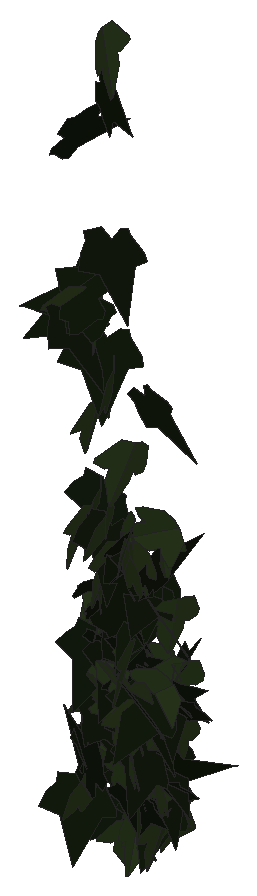
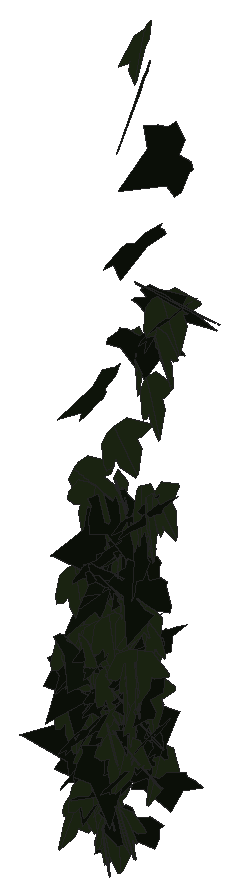
# SketchUp Ruby script. Lengths in inches.
U = 1.inch
M = Sketchup.active_model
def pt(a) = Geom::Point3d.new(a.map { |v| v * U })
def face(e, loops, mat)
  f = e.add_face(loops[0].map { |a| pt(a) })
  loops[1..].each { |l| e.add_face(l.map { |a| pt(a) }).erase! }
  f.material = f.back_material = mat if mat
  f
end
# faces: each face lists its corners as indices into pts; further lists are holes
def faces(e, pts, list, mat = nil) = list.each { |f| face(e, (f[0].is_a?(Array) ? f : [f]).map { |l| l.map { |i| pts[i] } }, mat) }
# xy, xz, yz: faces in a plane at the given z, y or x. An outline is a flat list of corners, or four numbers for a rectangle; further outlines are holes
def ring(l) = l.size == 4 ? [[l[0], l[1]], [l[2], l[1]], [l[2], l[3]], [l[0], l[3]]] : l.each_slice(2).to_a
def flat(e, list, mat, &to3) = list.each { |f| face(e, (f[0].is_a?(Array) ? f : [f]).map { |l| ring(l).map { |u, v| to3.(u, v) } }, mat) }
def xy(e, z, list, mat = nil) = flat(e, list, mat) { |x, y| [x, y, z] }
def xz(e, y, list, mat = nil) = flat(e, list, mat) { |x, z| [x, y, z] }
def yz(e, x, list, mat = nil) = flat(e, list, mat) { |y, z| [x, y, z] }
def lines(e, pts, list) = list.each { |a, b| e.add_line(pt(pts[a]), pt(pts[b])) }
# prism: a flat outline (further loops are holes) pulled along v
def prism(e, loops, v, mat = nil)
  f = face(e, loops, mat); d = Geom::Vector3d.new(v.map { |x| x * U })
  f.pushpull(f.normal.samedirection?(d) ? d.length : -d.length)
end
def box(e, o, s, mat = nil) = prism(e, [[o, [o[0] + s[0], o[1], o[2]], [o[0] + s[0], o[1] + s[1], o[2]], [o[0], o[1] + s[1], o[2]]]], [0, 0, s[2]], mat)
def at(x, y, z, deg = 0) = Geom::Transformation.translation(pt([x, y, z])) * Geom::Transformation.rotation(ORIGIN, Z_AXIS, deg.degrees)
def axes(o, x, y, z) = Geom::Transformation.new([*x, 0, *y, 0, *z, 0, *pt(o).to_a, 1])
def part(name) = M.definitions.add(name)
# library, detail: a bought-in or finely detailed component or shape, given as its bounding box
def library(name, o, s) = part(name).tap { |d| box(d.entities, o, s) }
def detail(e, o, s) = box(e.add_group.entities, o, s)
def put(e, d, t, mat = nil) = e.add_instance(d, t).tap { |i| i.material = mat if mat }
def group(e, t, mat = nil) = e.add_group.tap { |g| g.transformation = t; g.material = mat if mat }.entities
root = M.entities
M.materials.add("efeu1").color = [18, 25, 13]
M.materials.add("efeu2").color = [43, 57, 29]
c1 = part("ivyleaf_10")
p = [[0,0.5,-0.03],[-0.0625,2.02,-0.43],[-0.19,2.01,-0.46],[-0.54,1.05,-0.29],[-0.52,0.625,-0.18],[-0.83,0.76,-0.28],
  [-1.16,0.64,-0.33],[-1.15,0.33,-0.24],[-0.77,-0.39,0.02],[-0.3,-0.51,0.16],[0.04,-0.48,0.23],[-0.02,2.01,-0.4375],
  [-0.06,2.01,-0.43],[0.04,-0.49,0.23],[0.67,-0.49,0.14],[1.38,0.36,-0.2],[1.375,0.51,-0.24],[0.81,0.65,-0.19],
  [0.62,0.59,-0.15],[0.6,1.09,-0.28],[0.5,1.23,-0.31]]
faces(c1.entities,p,[[0,1,2,3,4,5,6,7,8,9,10],[11,12,0,13,14,15,16,17,18,19,20]],"efeu2")
c2 = part("ivyleaf_9")
p = [[1.54,2.16,1.25],[1.36,2.04,1.19],[-0.21,0.99,0.68],[-0.71,1.11,0.82],[-0.85,0.86,0.67],[-0.8,0.17,0.21],
  [-0.9,-0.01,0.1],[-0.67,-0.16,-0.02],[-0.08,-0.08,-0.05],[-0.03,-0.6,-0.4],[0.65,-0.88,-0.66],[0.83,-0.6,-0.49],
  [1.29,-0.42,-0.43],[1.8125,-0.07,-0.26],[1.21,0.44,0.15]]
faces(c2.entities,p,[[0,1,2,3,4,5,6,7,8,9,10,11,12,13,14]],"efeu1")
put(root,c1,axes([541.64,132.27,226.93],[-0.32026,-0.86998,0.20243],[-0.08974,-0.18262,-0.92683],[0.8887,-0.33195,-0.02065]))
put(root,c1,axes([541.54,132.71,225.9],[0.78925,-0.47005,-0.20203],[-0.14106,0.15709,-0.91657],[0.49179,0.79941,0.06132]))
put(root,c2,axes([541.35,132.85,207.7],[-0.47891,-0.67172,-0.25991],[0.19866,0.17682,-0.82303],[0.69231,-0.5154,0.05637]))
put(root,c1,axes([541.64,133.93,212.93],[-0.72073,-0.4905,0.00951],[0.0309,-0.06226,-0.86908],[0.48961,-0.7181,0.06886]))
put(root,c1,axes([541.52,134.76,206.88],[0.64822,-0.5421,0.01637],[0.01224,-0.01088,-0.84502],[0.5422,0.64834,-0.00049]))
put(root,c1,axes([541.65,133.19,211.51],[-0.09073,-0.85028,-0.01671],[0.00087,0.01671,-0.85511],[0.85045,-0.09073,-0.0009]))
put(root,c2,axes([541.25,133.23,209.89],[0.53426,-0.47664,-0.49908],[-0.2064,0.49191,-0.69074],[0.65853,0.54087,0.18841]))
put(root,c1,axes([541.63,133.15,218.88],[0.36674,-0.81694,-0.21878],[-0.0264,0.22729,-0.89297],[0.84532,0.36153,0.06703]))
put(root,c1,axes([541.69,133.99,210.95],[-0.3938,0.77477,0.0623],[-0.19432,-0.03052,-0.84884],[-0.75258,-0.39752,0.18658]))
put(root,c1,axes([541.23,133.61,214.32],[0.7081,-0.28038,0.42554],[0.41728,-0.09916,-0.7597],[0.29252,0.82016,0.05362]))
put(root,c2,axes([541.73,133.15,215.86],[0.28251,0.81104,0.16092],[-0.02124,0.17712,-0.85538],[-0.82658,0.27264,0.07698]))
put(root,c2,axes([541.42,131.87,233.13],[0.36103,0.55969,0.69828],[0.40169,0.57149,-0.66576],[-0.79968,0.53975,-0.01917]))
put(root,c1,axes([541.7,134.55,209.64],[-0.83966,-0.17869,-0.05465],[0.05299,0.01358,-0.85846],[0.17919,-0.84133,-0.00224]))
put(root,c2,axes([542.4,132.08,227.21],[-0.77918,0.34542,0.40853],[-0.47121,-0.10136,-0.81303],[-0.25332,-0.87393,0.25577]))
put(root,c1,axes([541.74,132.3125,208.3],[-0.04652,-0.72628,-0.52307],[0.05961,0.5201,-0.72746],[0.89304,-0.07255,0.02131]))
put(root,c2,axes([541.58,133.1875,208.68],[0.08281,-0.22127,0.85612],[0.45325,0.74893,0.14972],[-0.75925,0.42296,0.18276]))
put(root,c2,axes([542.27,132.29,227.06],[-0.86557,-0.19065,0.32604],[-0.31473,-0.08657,-0.88618],[0.20879,-0.92088,0.01581]))
put(root,c1,axes([541.81,133.7,212.51],[0.45582,-0.73664,-0.18739],[-0.00413,0.2161,-0.85954],[0.76009,0.44293,0.10771]))
put(root,c2,axes([541.36,134.35,206.7],[-0.10384,-0.39536,-0.73817],[0.38567,0.63766,-0.39578],[0.74328,-0.3861,0.10223]))
put(root,c2,axes([541.61,133.67,218.73],[-0.199,-0.81888,0.29676],[0.03297,-0.31127,-0.83681],[0.87037,-0.17544,0.09955]))
put(root,c2,axes([541.71,133.16,213.27],[-0.26657,-0.81591,0.24377],[-0.01935,-0.24957,-0.85646],[0.85133,-0.26115,0.05686]))
put(root,c2,axes([541.38,133.9375,209.84],[0.83919,-0.16882,0.03563],[0.03189,-0.02215,-0.85586],[0.16956,0.83965,-0.01541]))
put(root,c1,axes([541.96,133.86,212.31],[0.10595,-0.78561,-0.3752],[-0.01939,0.37575,-0.79222],[0.87039,0.104,0.02802]))
put(root,c2,axes([542.2,134.16,209.66],[-0.80552,0.2288,-0.18474],[0.16416,-0.09712,-0.83604],[-0.24399,-0.8207,0.04743]))
put(root,c2,axes([541.53,134.37,208.58],[0.18246,-0.80067,-0.25157],[0.00667,0.25883,-0.81891],[0.83923,0.17202,0.06121]))
put(root,c1,axes([541.82,134.63,206.85],[0.83582,-0.05974,-0.04926],[-0.0495,-0.00152,-0.83794],[0.05955,0.83727,-0.00503]))
put(root,c1,axes([541.52,133.75,214.92],[0.68119,0.29451,0.46585],[0.32645,0.38113,-0.7183],[-0.44406,0.73197,0.18657]))
put(root,c1,axes([541.91,132.17,218.6875],[0.25139,-0.80054,0.33629],[0.11256,-0.3171,-0.83901],[0.86098,0.2752,0.0115]))
put(root,c2,axes([541.5625,132.04,226.36],[0.2861,-0.8721,-0.29312],[-0.02299,0.30009,-0.91528],[0.91975,0.27877,0.0683]))
put(root,c2,axes([542.47,131.94,208.97],[0.0684,-0.1847,0.92206],[-0.46795,0.79522,0.19401],[-0.81568,-0.4717,-0.03398]))
put(root,c1,axes([542.31,133.54,211.69],[0.41356,0.45844,-0.60027],[-0.47931,-0.36961,-0.6125],[-0.58373,0.62828,0.07767]))
put(root,c1,axes([542.5,133.32,209.31],[0.20113,0.06766,-0.86768],[-0.45546,0.76704,-0.04577],[0.74161,0.45273,0.20721]))
put(root,c1,axes([542.24,134.24,206.02],[-0.4347,-0.70588,0.01715],[-0.00974,-0.01415,-0.82899],[0.70602,-0.43481,-0.00087]))
put(root,c2,axes([541.42,133.55,211.33],[0.58731,-0.20498,0.58914],[0.61661,0.06847,-0.59087],[0.09428,0.82905,0.19446]))
put(root,c1,axes([542.41,133.23,214.73],[-0.94377,-0.01712,0.07843],[-0.0784,-0.00235,-0.94392],[0.01726,-0.94702,0.00092]))
put(root,c2,axes([542.98,133.19,210.46],[-0.5526,0.53484,0.54174],[-0.42871,0.33455,-0.76759],[-0.62909,-0.6978,0.04722]))
put(root,c2,axes([542.33,132.8125,213.78],[0.6793,0.37606,-0.39581],[-0.37034,-0.14687,-0.77512],[-0.40117,0.77236,0.04533]))
put(root,c1,axes([542.15,133.86,212.04],[0.46357,-0.70071,0.2164],[0.24367,-0.09429,-0.82731],[0.69169,0.50283,0.14642]))
put(root,c1,axes([542.43,132.07,223.11],[0.16423,-0.91899,-0.00136],[0.0056,0.00238,-0.93354],[0.91898,0.16422,0.00593]))
put(root,c2,axes([542.07,133.24,211.15],[0.13626,-0.66652,-0.62668],[-0.07693,0.623,-0.67933],[0.91162,0.1522,0.03634]))
put(root,c1,axes([542.33,134.43,209.9375],[0.46105,-0.71773,0.13539],[0.10515,-0.09321,-0.85222],[0.72278,0.47139,0.03762]))
put(root,c1,axes([542.41,134.77,206.05],[0.47635,-0.69796,-0.05806],[0.04799,0.10258,-0.83941],[0.69873,0.46879,0.09723]))
put(root,c2,axes([541.86,133.6875,216.19],[0.27149,-0.43402,0.79329],[0.37499,-0.69966,-0.51113],[0.82284,0.46205,-0.0288]))
put(root,c2,axes([542.78,134.28,208.62],[-0.02172,0.85905,-0.06341],[-0.0085,-0.06364,-0.85927],[-0.86135,-0.02103,0.01008]))
put(root,c1,axes([542.65,134.18,212],[-0.06434,-0.8658,0.10447],[-0.03045,-0.10246,-0.86789],[0.87154,-0.0675,-0.02261]))
put(root,c1,axes([543.22,132.7,209.41],[0.05243,0.20816,0.87879],[-0.89821,0.10359,0.02905],[-0.09395,-0.87424,0.21269]))
put(root,c1,axes([542.65,132.25,218.61],[0.18382,-0.86777,-0.30896],[0.01184,0.31725,-0.88402],[0.92106,0.16911,0.07302]))
put(root,c1,axes([542.57,134.14,210.5],[-0.33148,0.80212,0.11016],[-0.05778,0.09529,-0.86775],[-0.80758,-0.33606,0.01687]))
put(root,c1,axes([542.53,134.49,206.19],[0.08963,-0.82463,0.07011],[0.23249,-0.04259,-0.79818],[0.79428,0.10552,0.22572]))
put(root,c2,axes([542.24,133.7,213.52],[0.36119,-0.79465,-0.00055],[0.00007,0.00063,-0.87288],[0.79465,0.36119,0.00032]))
put(root,c1,axes([542.97,131.6,215.8],[0.092,-0.22957,-0.878],[-0.31309,0.82029,-0.24729],[0.8518,0.3263,0.00394]))
put(root,c1,axes([542.8125,133.9,213.94],[-0.24172,-0.85367,0.03783],[0.0061,-0.04104,-0.88707],[0.85448,-0.24119,0.01704]))
put(root,c1,axes([542.76,134.19,206.67],[0.52905,-0.65103,-0.10714],[-0.0624,0.08734,-0.83886],[0.65683,0.53268,0.0066]))
put(root,c2,axes([542.63,134.18,211.65],[-0.37296,-0.79026,-0.03407],[0.03406,0.02158,-0.87358],[0.79026,-0.37389,0.02158]))
put(root,c2,axes([542.57,132.49,225.46],[-0.56469,-0.64212,-0.4449],[0.31985,0.3108,-0.85453],[0.71271,-0.64824,0.03099]))
put(root,c2,axes([542.83,132.02,216.04],[0.22033,0.76144,0.49287],[0.10775,0.48164,-0.79226],[-0.90062,0.24391,0.02579]))
put(root,c1,axes([542.88,133.12,216.08],[0.245,-0.76909,-0.39565],[-0.08234,0.38861,-0.8064],[0.86097,0.25603,0.03547]))
put(root,c1,axes([542.84,132.85,213.03],[0.45609,-0.62,-0.44837],[-0.0652,0.4886,-0.74194],[0.76235,0.41272,0.20479]))
put(root,c2,axes([542.53,133.13,212.875],[-0.06933,-0.77836,0.50808],[0.03061,-0.51112,-0.77885],[0.929,-0.04125,0.06358]))
put(root,c2,axes([542.57,132.74,218.1875],[-0.04367,-0.90714,0.04068],[-0.0068,-0.0404,-0.90818],[0.90803,-0.04393,-0.00484]))
put(root,c2,axes([542.57,134.08,210.625],[0.09051,-0.85614,-0.00431],[-0.01489,0.00276,-0.86079],[0.85602,0.09057,-0.01451]))
put(root,c1,axes([542.83,132.3,217.52],[0.24872,-0.77204,0.41701],[0.18079,-0.37906,-0.80959],[0.85864,0.30345,0.04966]))
put(root,c1,axes([543.41,133.02,210.52],[-0.43908,0.34645,0.68714],[-0.66205,0.23321,-0.54063],[-0.39227,-0.78139,0.1433]))
put(root,c2,axes([542.68,134.08,211.29],[-0.01145,-0.87439,-0.09647],[-0.00422,0.09654,-0.87445],[0.87969,-0.01091,-0.00545]))
put(root,c1,axes([542.96,132.75,216.66],[-0.87294,0.16843,-0.07553],[0.07749,0.00302,-0.88886],[-0.16754,-0.87619,-0.01758]))
put(root,c2,axes([542.99,131.78,235.7],[0.57234,-0.31792,-0.72658],[-0.62067,0.37824,-0.65441],[0.49372,0.84405,0.01959]))
put(root,c1,axes([542.9375,133.73,206.62],[0.12831,0.75026,-0.38641],[-0.04867,-0.38362,-0.761],[-0.84252,0.13642,-0.01488]))
put(root,c1,axes([542.88,134.16,211.78],[0.77811,0.40461,0.02343],[0.01679,0.01849,-0.87698],[-0.40494,0.77824,0.00866]))
put(root,c2,axes([543.5,133.61,215.35],[-0.86136,0.18451,0.04284],[-0.03667,0.03324,-0.88055],[-0.18584,-0.86178,-0.02479]))
put(root,c1,axes([542.51,132.29,212.64],[-0.50233,0.10722,-0.7816],[0.7744,-0.10996,-0.51279],[-0.15067,-0.92258,-0.02972]))
put(root,c1,axes([543.2,134.57,207.42],[-0.49091,-0.69208,0.11224],[0.02117,-0.15159,-0.8421],[0.7008,-0.48022,0.10406]))
put(root,c2,axes([542.8,132.52,229.26],[0.11012,-0.92285,-0.20654],[-0.01177,0.20658,-0.92932],[0.94561,0.11004,0.01249]))
put(root,c1,axes([543.1,131.81,237.36],[-0.1917,0.96324,-0.01831],[-0.06293,-0.03114,-0.97979],[-0.96136,-0.19003,0.06778]))
put(root,c1,axes([543.25,132.875,221.23],[-0.20463,-0.8275,0.37986],[0.04621,-0.39827,-0.84272],[0.90935,-0.16597,0.1283]))
put(root,c2,axes([543.66,133.85,215.91],[-0.85923,-0.01561,0.18594],[-0.18372,-0.08243,-0.85589],[0.03263,-0.87525,0.07729]))
put(root,c2,axes([543.56,132.82,218.33],[-0.18755,0.80911,-0.30417],[0.01054,-0.30909,-0.82868],[-0.86433,-0.17934,0.0559]))
put(root,c1,axes([543.38,133.52,213.41],[-0.62529,-0.61241,0.15654],[-0.01797,-0.20289,-0.86548],[0.63185,-0.61183,0.13031]))
put(root,c1,axes([543.6875,132.39,212.02],[-0.7803,-0.24032,-0.53592],[-0.51307,-0.15483,0.81647],[-0.28587,0.93387,-0.00254]))
put(root,c2,axes([543.17,134.61,207.16],[-0.33399,-0.78503,0.02418],[0.02725,-0.03785,-0.85219],[0.78492,-0.33272,0.03988]))
put(root,c2,axes([543.67,133.06,211.56],[-0.52115,0.71131,-0.10396],[0.07122,-0.07669,-0.88171],[-0.71533,-0.52586,-0.01204]))
put(root,c1,axes([543.34,131.76,224.63],[0.40503,-0.7941,-0.26058],[-0.019,0.28075,-0.88508],[0.83554,0.39132,0.10619]))
put(root,c2,axes([543.29,133.75,215.11],[-0.4702,-0.7567,0.0819],[0.02797,-0.11339,-0.88699],[0.76061,-0.46361,0.08325]))
put(root,c2,axes([543.29,132.68,215.08],[0.73391,-0.03562,-0.48159],[-0.48081,0.02773,-0.73476],[0.04499,0.87738,0.00367]))
put(root,c1,axes([543.62,133.01,209.41],[0.69849,-0.30919,-0.4814],[-0.40549,0.26845,-0.76076],[0.40364,0.80472,0.06882]))
put(root,c2,axes([543.27,132.33,213.01],[-0.08446,0.36952,-0.82506],[-0.18773,0.80342,0.37904],[0.88432,0.20585,0.00167]))
put(root,c2,axes([543.55,132.18,215.37],[0.23649,0.58446,0.62609],[-0.64208,-0.30889,0.53088],[0.56684,-0.59372,0.34013]))
put(root,c1,axes([543.73,132.65,217.87],[-0.81637,0.30529,0.21632],[-0.23253,-0.00721,-0.86737],[-0.29313,-0.84451,0.0856]))
put(root,c2,axes([543.62,133.68,208.16],[0.5197,0.64386,-0.22357],[-0.1824,-0.1395,-0.82577],[-0.65671,0.54828,0.05243]))
put(root,c2,axes([543.05,133.97,213],[0.64422,-0.60844,-0.01915],[0.07575,0.1078,-0.87649],[0.60401,0.63543,0.13035]))
put(root,c1,axes([544.07,131.92,217.77],[-0.59698,0.32987,0.60549],[-0.58693,0.1772,-0.67522],[-0.36186,-0.83162,0.0963]))
put(root,c1,axes([543.67,134.81,206.6],[-0.04342,-0.54945,-0.64357],[0.04071,0.64232,-0.55113],[0.84524,-0.05916,-0.00651]))
put(root,c1,axes([543.71,132.71,208.24],[0.52231,-0.52607,-0.47161],[-0.08302,0.53672,-0.69065],[0.70162,0.45513,0.26935]))
put(root,c1,axes([543.69,132.29,218.69],[0.53044,-0.7408,-0.01632],[-0.00936,0.01337,-0.91112],[0.74092,0.53052,0.00017]))
put(root,c2,axes([543.48,133.78,216.46],[-0.08356,-0.87928,0.04149],[-0.00628,-0.04108,-0.88324],[0.88024,-0.08377,-0.00236]))
put(root,c1,axes([543.82,134.22,212.95],[0.63776,-0.52621,-0.27544],[-0.15654,0.24094,-0.82277],[0.57294,0.65158,0.0818]))
put(root,c1,axes([543.85,132.45,211.87],[-0.10606,-0.89547,0.25789],[-0.00413,-0.2591,-0.90138],[0.93186,-0.10306,0.02536]))
put(root,c2,axes([543.85,132.29,208.59],[0.64016,0.26012,-0.52154],[-0.49577,-0.16425,-0.69044],[-0.3064,0.80922,0.0275]))
put(root,c2,axes([544.05,134.16,212.39],[0.08121,0.58589,0.6476],[-0.13844,0.65081,-0.57143],[-0.86226,-0.0493,0.15274]))
put(root,c1,axes([543.91,134.01,211.2],[-0.47219,-0.71255,0.14671],[-0.01958,-0.16239,-0.85174],[0.72723,-0.46703,0.07232]))
put(root,c1,axes([543.74,132.56,209.89],[-0.45354,0.78711,-0.00919],[0.00109,-0.00998,-0.90842],[-0.78716,-0.45352,0.00404]))
put(root,c2,axes([543.49,133.57,215.49],[0.86945,-0.26156,-0.28108],[-0.26972,0.07912,-0.90794],[0.27325,0.91033,-0.00185]))
put(root,c2,axes([543.4,133.69,211.3],[0.44867,-0.74076,0.03737],[0.0165,-0.03369,-0.86604],[0.74152,0.44896,-0.00334]))
put(root,c2,axes([543.59,133.39,216.02],[-0.23142,-0.75339,0.43693],[0.21856,-0.48787,-0.72545],[0.84305,-0.08033,0.30801]))
put(root,c1,axes([543.95,132.44,209.91],[-0.2882,0.74799,0.43423],[-0.18418,0.39413,-0.80115],[-0.84506,-0.341,0.02652]))
put(root,c1,axes([543.76,132.17,214.14],[0.43185,-0.69209,0.40773],[0.21396,-0.34708,-0.81577],[0.77425,0.48194,-0.00198]))
put(root,c2,axes([543.59,134.46,208.32],[0.18327,-0.84035,0.05099],[-0.00173,-0.05256,-0.86001],[0.8419,0.18282,-0.01287]))
put(root,c2,axes([543.64,134.26,209.57],[0.24494,-0.78538,-0.25499],[-0.02906,0.2576,-0.82136],[0.82523,0.24219,0.04676]))
put(root,c1,axes([544.01,133.66,208.6],[-0.29008,0.77639,0.22455],[-0.11351,0.19708,-0.82802],[-0.8002,-0.3094,0.03605]))
put(root,c1,axes([544.05,133.6,207.14],[0.14065,-0.87751,0.16074],[0.02287,-0.15913,-0.88871],[0.89182,0.14248,-0.00256]))
put(root,c2,axes([543.8125,133.81,211.89],[0.70521,0.52338,0.11083],[0.08173,0.07583,-0.87812],[-0.5287,0.70983,0.01209]))
put(root,c2,axes([544.19,133.72,211.6],[0.52243,0.59745,-0.33857],[-0.31411,-0.1704,-0.78538],[-0.61067,0.59877,0.11432]))
put(root,c2,axes([543.96,133,216.47],[0.13341,0.24727,0.91679],[0.4697,0.78742,-0.28073],[-0.82525,0.48815,-0.01157]))
put(root,c2,axes([543.45,132.43,212.66],[0.49075,-0.58891,0.47638],[0.35106,-0.32615,-0.76484],[0.6712,0.60117,0.05173]))
put(root,c2,axes([543.93,132.9375,210.02],[-0.08215,-0.82556,0.30845],[-0.04139,-0.30583,-0.82957],[0.88033,-0.09142,-0.01022]))
put(root,c1,axes([544.3,134.2,210.35],[-0.21367,-0.8455,-0.05609],[0.02186,0.05233,-0.87204],[0.84708,-0.21462,0.00836]))
put(root,c2,axes([543.92,134.22,211.95],[0.0503,-0.87118,0.02439],[-0.00066,-0.02447,-0.87263],[0.87152,0.05026,-0.00207]))
put(root,c2,axes([543.68,133.3125,223.27],[0.66095,-0.63081,-0.07012],[0.0605,0.1634,-0.89963],[0.63181,0.64426,0.1595]))
put(root,c1,axes([544.25,133.27,218.62],[-0.86318,0.17521,-0.08906],[0.05329,-0.17745,-0.86567],[-0.18918,-0.84943,0.16247]))
put(root,c1,axes([544.7,132.77,212.78],[0.57988,0.04419,-0.70175],[-0.70181,0.09223,-0.57413],[0.04318,0.90566,0.09271]))
put(root,c1,axes([544.38,134.125,212.74],[-0.39491,-0.78033,0.06766],[0.0286,-0.09009,-0.87207],[0.78273,-0.39041,0.066]))
put(root,c1,axes([544.33,134.08,212.76],[-0.06647,-0.66066,0.57596],[0.09716,-0.57961,-0.65363],[0.87107,0.01424,0.11685]))
put(root,c2,axes([544.45,132.67,212.3],[-0.6021,-0.62334,0.08925],[-0.05824,-0.06783,-0.86663],[0.627,-0.60489,0.00521]))
put(root,c2,axes([543.68,133.86,208.79],[0.47721,-0.00913,0.77376],[0.75253,0.21722,-0.46156],[-0.18024,0.88275,0.12158]))
put(root,c1,axes([544.94,132.7,218.99],[0.42561,0.09275,-0.80304],[-0.80471,0.13493,-0.41091],[0.07689,0.89878,0.14455]))
put(root,c1,axes([544.5,133.77,215.38],[-0.31589,-0.83319,0.06967],[0.01228,-0.07909,-0.89019],[0.836,-0.31366,0.0394]))
